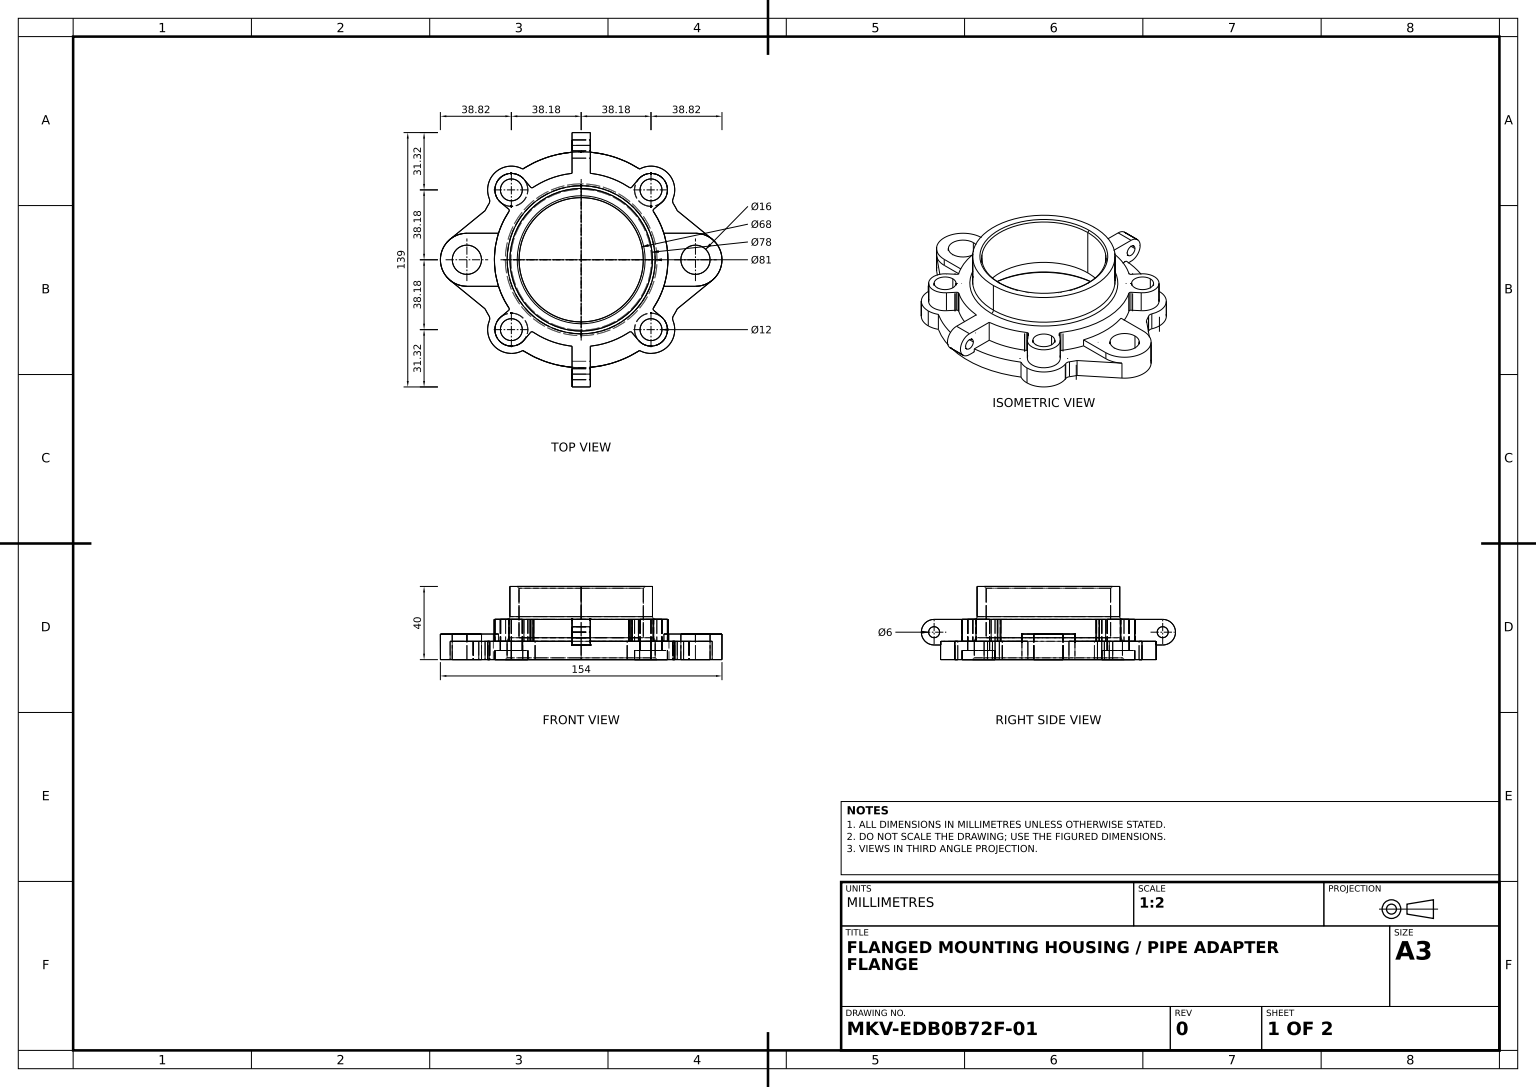
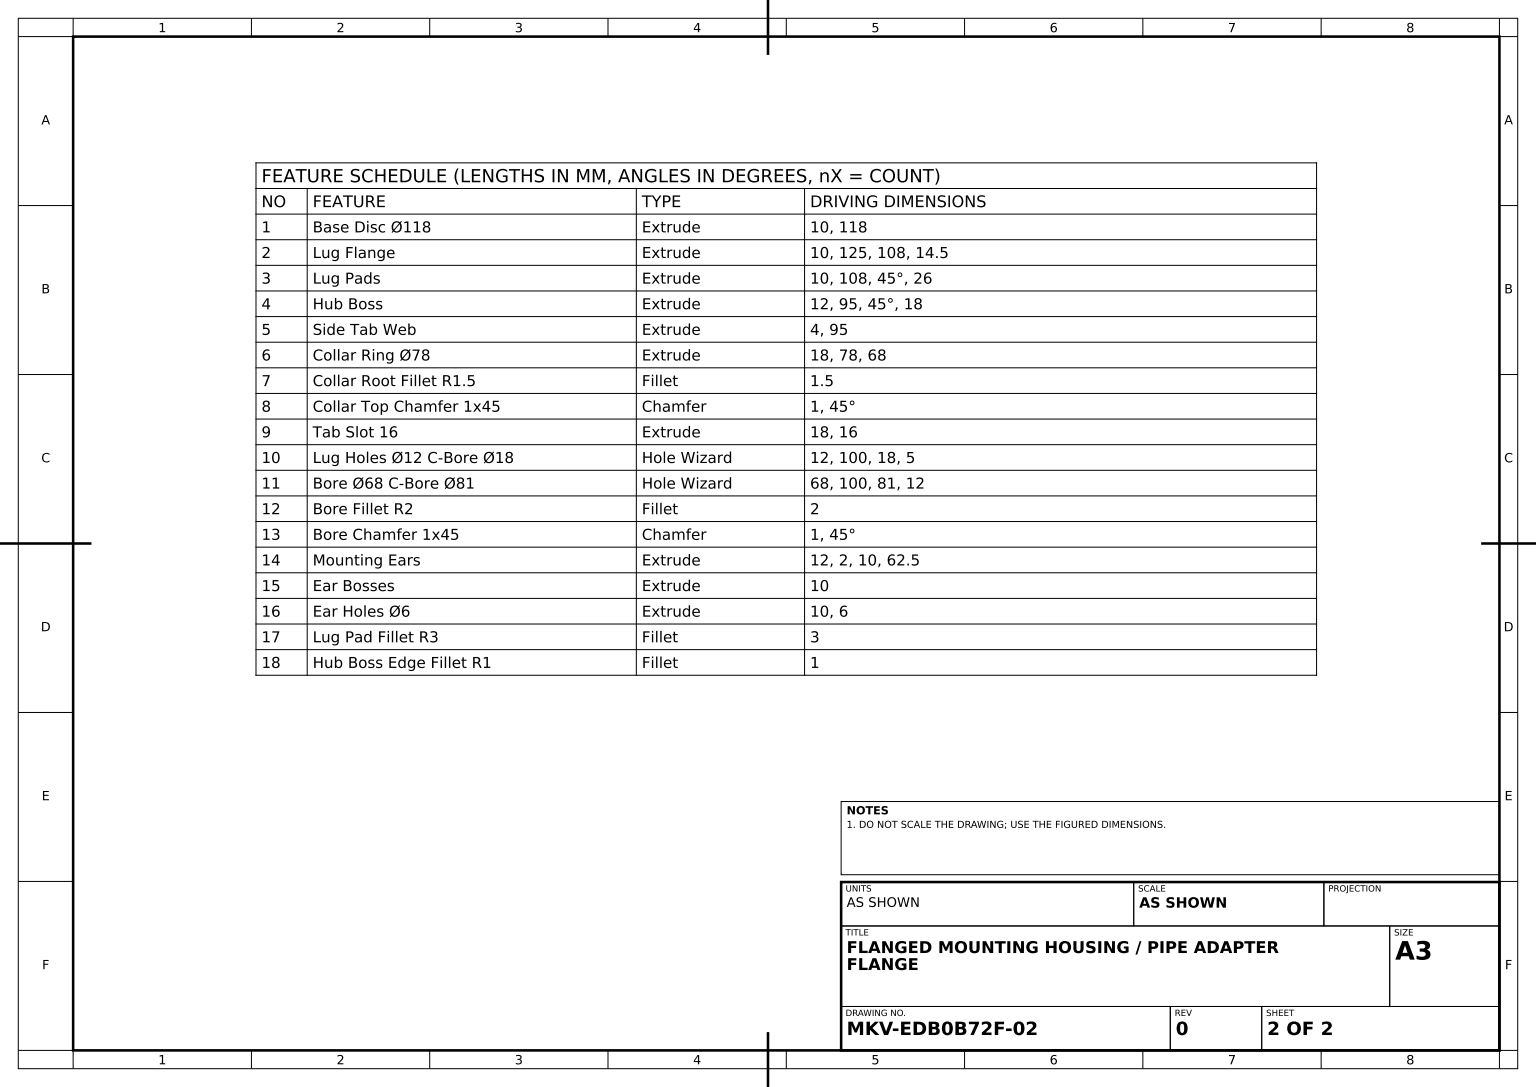
solid
v1 (-62.5,14,-14.5)
v2 (-62.5,10,-14.5)
e1 v1 v2 LINE
v3 (-45.232732,14,-14.5)
e2 v3 v1 LINE
v4 (-45.232732,10,-14.5)
e3 v3 v4 LINE
e4 v4 v2 LINE
face PLANE(AX(P(-62.5,14,-14.5),D(0,0,1),D(1,0,0))) rev [-e1 -e2 e3 e4]
v5 (5,8,-62.5)
v6 (5,15,-69.5)
e5 v5 v6 CIRCLE(AX(P(5,15,-62.5),D(1,0,0),D(0,0,-1)),7)
v7 (-5,8,-62.5)
e6 v5 v7 LINE
v8 (-5,15,-69.5)
e7 v7 v8 CIRCLE(AX(P(-5,15,-62.5),D(1,0,0),D(0,0,-1)),7)
e8 v8 v6 LINE
face CYL(AX(P(-5,15,-62.5),D(1,0,0),D(0,0,-1)),7) [-e5 e6 e7 e8]
v9 (71.664,10,-11.237042)
v10 (71.664,0,-11.237042)
e9 v9 v10 LINE
v11 (62.5,10,-14.5)
e10 v9 v11 CIRCLE(AX(P(62.5,10,0),D(0,1,0),D(0,0,-1)),14.5)
v12 (62.5,14,-14.5)
e11 v12 v11 LINE
v13 (62.5,14,14.5)
e12 v13 v12 CIRCLE(AX(P(62.5,14,0),D(0,1,0),D(0,0,-1)),14.5)
v14 (62.5,10,14.5)
e13 v13 v14 LINE
v15 (71.664,10,11.237042)
e14 v14 v15 CIRCLE(AX(P(62.5,10,0),D(0,1,0),D(0,0,-1)),14.5)
v16 (71.664,0,11.237042)
e15 v15 v16 LINE
e16 v10 v16 CIRCLE(AX(P(62.5,0,0),D(0,-1,0),D(0,0,-1)),14.5)
face CYL(AX(P(62.5,10,0),D(0,-1,0),D(0,0,-1)),14.5) [-e9 e10 -e11 -e12 e13 e14 e15 -e16]
v17 (45.232732,14,14.5)
e17 v17 v13 LINE
v18 (45.232732,10,14.5)
e18 v17 v18 LINE
e19 v18 v14 LINE
face PLANE(AX(P(62.5,14,14.5),D(0,0,-1),D(-1,0,0))) rev [-e13 -e17 e18 e19]
v19 (-38.183766,22,32.183766)
v20 (-38.183766,5,32.183766)
e20 v19 v20 LINE
v21 (-38.183766,5,44.183766)
e21 v20 v21 CIRCLE(AX(P(-38.183766,5,38.183766),D(0,-1,0),D(0,0,-1)),6)
v22 (-38.183766,22,44.183766)
e22 v22 v21 LINE
e23 v19 v22 CIRCLE(AX(P(-38.183766,22,38.183766),D(0,-1,0),D(0,0,-1)),6)
face CYL(AX(P(-38.183766,0,38.183766),D(0,-1,0),D(0,0,-1)),6) rev [e20 e21 -e22 -e23]
v23 (-5,8,58.787754)
v24 (-5,8,62.5)
e24 v23 v24 LINE
v25 (5,8,58.787754)
e25 v23 v25 CIRCLE(AX(P(0,8,0),D(0,1,0),D(0,0,1)),59)
v26 (5,8,62.5)
e26 v26 v25 LINE
e27 v24 v26 LINE
face PLANE(AX(P(0,8,0),D(0,1,0),D(0,0,1))) rev [-e24 e25 -e26 -e27]
v27 (-5,15,-59.5)
v28 (-5,15,-65.5)
e28 v27 v28 CIRCLE(AX(P(-5,15,-62.5),D(1,0,0),D(0,0,-1)),3)
v29 (5,15,-59.5)
e29 v27 v29 LINE
v30 (5,15,-65.5)
e30 v29 v30 CIRCLE(AX(P(5,15,-62.5),D(1,0,0),D(0,0,-1)),3)
e31 v28 v30 LINE
face CYL(AX(P(-5,15,-62.5),D(1,0,0),D(0,0,-1)),3) rev [-e28 e29 e30 -e31]
v31 (-50.441848,10,-30.604247)
v32 (-50.441848,0,-30.604247)
e32 v31 v32 LINE
v33 (-52.548788,0,-26.825824)
e33 v32 v33 CIRCLE(AX(P(0,0,0),D(0,1,0),D(0,0,1)),59)
v34 (-52.548788,10,-26.825824)
e34 v34 v33 LINE
e35 v31 v34 CIRCLE(AX(P(0,10,0),D(0,1,0),D(0,0,1)),59)
face CYL(AX(P(0,10,0),D(0,-1,0),D(0,0,-1)),59) [e32 e33 -e34 -e35]
v35 (-39.700135,10,27.679401)
v36 (-39.513984,10,26.360863)
e36 v35 v36 CIRCLE(AX(P(-40.345857,10,26.915829),D(0,1,0),D(0,0,1)),1)
v37 (-45.232732,10,14.5)
e37 v37 v36 CIRCLE(AX(P(0,10,0),D(0,1,0),D(0,0,1)),47.5)
v38 (-62.5,10,14.5)
e38 v38 v37 LINE
v39 (-71.664,10,11.237042)
e39 v39 v38 CIRCLE(AX(P(-62.5,10,0),D(0,1,0),D(0,0,1)),14.5)
v40 (-52.548788,10,26.825824)
e40 v40 v39 LINE
v41 (-50.441848,10,30.604247)
e41 v40 v41 CIRCLE(AX(P(0,10,0),D(0,1,0),D(0,0,1)),59)
v42 (-50.22739,10,33.289778)
e42 v41 v42 CIRCLE(AX(P(-53.006688,10,32.160396),D(0,-1,0),D(0,0,1)),3)
v43 (-38.183766,10,51.183766)
e43 v42 v43 CIRCLE(AX(P(-38.183766,10,38.183766),D(0,1,0),D(0,0,1)),13)
v44 (-31.95732,10,49.595662)
e44 v43 v44 CIRCLE(AX(P(-38.183766,10,38.183766),D(0,1,0),D(0,0,1)),13)
v45 (-5,10,58.787754)
e45 v44 v45 CIRCLE(AX(P(0,10,0),D(0,1,0),D(0,0,1)),59)
v46 (-5,10,47.236109)
e46 v46 v45 LINE
v47 (-26.360863,10,39.513984)
e47 v47 v46 CIRCLE(AX(P(0,10,0),D(0,1,0),D(0,0,1)),47.5)
v48 (-26.915829,10,39.345857)
e48 v47 v48 CIRCLE(AX(P(-26.915829,10,40.345857),D(0,1,0),D(0,0,1)),1)
v49 (-27.679401,10,39.700135)
e49 v48 v49 CIRCLE(AX(P(-26.915829,10,40.345857),D(0,1,0),D(0,0,1)),1)
v50 (-31.311611,10,43.995262)
e50 v50 v49 LINE
v51 (-43.995262,10,31.311611)
e51 v51 v50 CIRCLE(AX(P(-38.183766,10,38.183766),D(0,1,0),D(0,0,-1)),9)
e52 v35 v51 LINE
face PLANE(AX(P(0,10,0),D(0,1,0),D(0,0,1))) [e36 -e37 -e38 -e39 -e40 e41 e42 e43 e44 e45 -e46 -e47 e48 e49 -e50 -e51 -e52]
v52 (38.183766,5,-29.183766)
v53 (38.183766,5,-47.183766)
e53 v52 v53 CIRCLE(AX(P(38.183766,5,-38.183766),D(0,-1,0),D(0,0,-1)),9)
v54 (38.183766,0,-29.183766)
e54 v52 v54 LINE
v55 (38.183766,0,-47.183766)
e55 v54 v55 CIRCLE(AX(P(38.183766,0,-38.183766),D(0,-1,0),D(0,0,-1)),9)
e56 v53 v55 LINE
face CYL(AX(P(38.183766,0,-38.183766),D(0,-1,0),D(0,0,-1)),9) rev [-e53 e54 e55 -e56]
v56 (0,0,-59)
v57 (-31.95732,0,-49.595662)
e57 v56 v57 CIRCLE(AX(P(0,0,0),D(0,1,0),D(0,0,1)),59)
v58 (-31.95732,10,-49.595662)
e58 v57 v58 LINE
v59 (-5,10,-58.787754)
e59 v59 v58 CIRCLE(AX(P(0,10,0),D(0,1,0),D(0,0,1)),59)
v60 (-5,8,-58.787754)
e60 v59 v60 LINE
v61 (0,8,-59)
e61 v60 v61 CIRCLE(AX(P(0,8,0),D(0,-1,0),D(0,0,-1)),59)
e62 v61 v56 LINE
face CYL(AX(P(0,10,0),D(0,-1,0),D(0,0,-1)),59) [e57 e58 -e59 e60 e61 e62]
v62 (38.183766,22,-47.183766)
v63 (38.183766,10,-47.183766)
e63 v62 v63 LINE
v64 (43.995262,22,-31.311611)
e64 v64 v62 CIRCLE(AX(P(38.183766,22,-38.183766),D(0,1,0),D(0,0,-1)),9)
v65 (43.995262,10,-31.311611)
e65 v64 v65 LINE
e66 v65 v63 CIRCLE(AX(P(38.183766,10,-38.183766),D(0,1,0),D(0,0,-1)),9)
face CYL(AX(P(38.183766,22,-38.183766),D(0,-1,0),D(0,0,-1)),9) [-e63 -e64 e65 e66]
v66 (38.183766,5,29.183766)
v67 (38.183766,0,29.183766)
e67 v66 v67 LINE
v68 (38.183766,5,47.183766)
e68 v68 v66 CIRCLE(AX(P(38.183766,5,38.183766),D(0,-1,0),D(0,0,-1)),9)
v69 (38.183766,0,47.183766)
e69 v68 v69 LINE
e70 v69 v67 CIRCLE(AX(P(38.183766,0,38.183766),D(0,-1,0),D(0,0,-1)),9)
face CYL(AX(P(38.183766,0,38.183766),D(0,-1,0),D(0,0,-1)),9) rev [-e67 -e68 e69 e70]
v70 (-50.22739,0,33.289778)
e71 v42 v70 LINE
v71 (-50.441848,0,30.604247)
e72 v71 v41 LINE
e73 v70 v71 CIRCLE(AX(P(-53.006688,0,32.160396),D(0,1,0),D(0,0,1)),3)
face CYL(AX(P(-53.006688,0,32.160396),D(0,-1,0),D(0,0,-1)),3) rev [-e71 -e42 -e72 -e73]
v72 (-38.183766,22,-47.183766)
v73 (-38.183766,10,-47.183766)
e74 v72 v73 LINE
v74 (-31.311611,22,-43.995262)
e75 v74 v72 CIRCLE(AX(P(-38.183766,22,-38.183766),D(0,1,0),D(0,0,1)),9)
v75 (-31.311611,10,-43.995262)
e76 v74 v75 LINE
e77 v75 v73 CIRCLE(AX(P(-38.183766,10,-38.183766),D(0,1,0),D(0,0,1)),9)
face CYL(AX(P(-38.183766,22,-38.183766),D(0,-1,0),D(0,0,-1)),9) [-e74 -e75 e76 e77]
v76 (45.232732,10,-14.5)
v77 (39.513984,10,-26.360863)
e78 v76 v77 CIRCLE(AX(P(0,10,0),D(0,1,0),D(0,0,1)),47.5)
v78 (39.513984,22,-26.360863)
e79 v77 v78 LINE
v79 (39.513984,22,26.360863)
e80 v79 v78 CIRCLE(AX(P(0,22,0),D(0,1,0),D(0,0,1)),47.5)
v80 (39.513984,10,26.360863)
e81 v79 v80 LINE
e82 v80 v18 CIRCLE(AX(P(0,10,0),D(0,1,0),D(0,0,1)),47.5)
v81 (45.232732,14,-14.5)
e83 v81 v17 CIRCLE(AX(P(0,14,0),D(0,-1,0),D(0,0,-1)),47.5)
e84 v81 v76 LINE
face CYL(AX(P(0,22,0),D(0,-1,0),D(0,0,-1)),47.5) [e78 e79 -e80 e81 e82 -e18 -e83 e84]
v82 (0,40,39)
v83 (0,23.5,39)
e85 v82 v83 LINE
v84 (0,23.5,-39)
e86 v83 v84 CIRCLE(AX(P(0,23.5,0),D(0,1,0),D(0,0,-1)),39)
v85 (0,40,-39)
e87 v85 v84 LINE
e88 v82 v85 CIRCLE(AX(P(0,40,0),D(0,1,0),D(0,0,1)),39)
face CYL(AX(P(0,40,0),D(0,-1,0),D(0,0,-1)),39) [e85 e86 -e87 -e88]
v86 (-26.360863,22,39.513984)
e89 v86 v47 LINE
v87 (-26.915829,22,39.345857)
e90 v87 v86 CIRCLE(AX(P(-26.915829,22,40.345857),D(0,-1,0),D(0,0,-1)),1)
e91 v87 v48 LINE
face CYL(AX(P(-26.915829,22,40.345857),D(0,-1,0),D(0,0,-1)),1) rev [-e89 -e90 e91 -e48]
v88 (31.95732,0,-49.595662)
e92 v88 v56 CIRCLE(AX(P(0,0,0),D(0,1,0),D(0,0,1)),59)
v89 (5,8,-58.787754)
e93 v61 v89 CIRCLE(AX(P(0,8,0),D(0,-1,0),D(0,0,-1)),59)
v90 (5,10,-58.787754)
e94 v89 v90 LINE
v91 (31.95732,10,-49.595662)
e95 v91 v90 CIRCLE(AX(P(0,10,0),D(0,1,0),D(0,0,1)),59)
e96 v88 v91 LINE
face CYL(AX(P(0,10,0),D(0,-1,0),D(0,0,-1)),59) [e92 -e62 e93 e94 -e95 -e96]
e97 v7 v60 LINE
e98 v89 v5 LINE
face PLANE(AX(P(0,8,0),D(0,-1,0),D(0,0,-1))) [-e61 -e97 -e6 -e98 -e93]
v92 (-5,22,-62.5)
e99 v8 v92 CIRCLE(AX(P(-5,15,-62.5),D(1,0,0),D(0,0,-1)),7)
v93 (5,22,-62.5)
e100 v93 v92 LINE
e101 v6 v93 CIRCLE(AX(P(5,15,-62.5),D(1,0,0),D(0,0,-1)),7)
face CYL(AX(P(-5,15,-62.5),D(1,0,0),D(0,0,-1)),7) [e99 -e100 -e101 -e8]
v94 (0,22,40.5)
e102 v94 v83 CIRCLE(AX(P(0,23.5,40.5),D(1,0,0),D(0,0,-1)),1.5)
v95 (0,22,-40.5)
e103 v95 v94 CIRCLE(AX(P(0,22,0),D(0,-1,0),D(0,0,-1)),40.5)
e104 v95 v84 CIRCLE(AX(P(0,23.5,-40.5),D(-1,0,0),D(0,0,1)),1.5)
face TORUS(AX(P(0,23.5,0),D(0,-1,0),D(0,0,-1)),40.5,1.5) rev [-e86 -e102 -e103 e104]
v96 (52.548788,10,26.825824)
v97 (52.548788,0,26.825824)
e105 v96 v97 LINE
e106 v16 v97 LINE
e107 v15 v96 LINE
face PLANE(AX(P(71.664,10,11.237042),D(0.632,0,0.774968386),D(0.774968386,0,-0.632))) [e105 -e106 -e15 e107]
e108 v55 v54 CIRCLE(AX(P(38.183766,0,-38.183766),D(0,-1,0),D(0,0,-1)),9)
e109 v53 v52 CIRCLE(AX(P(38.183766,5,-38.183766),D(0,-1,0),D(0,0,-1)),9)
face CYL(AX(P(38.183766,0,-38.183766),D(0,-1,0),D(0,0,-1)),9) rev [e56 e108 -e54 -e109]
v98 (0,12,38.5)
v99 (0,12,-38.5)
e110 v98 v99 CIRCLE(AX(P(0,12,0),D(0,-1,0),D(0,0,1)),38.5)
e111 v99 v98 CIRCLE(AX(P(0,12,0),D(0,-1,0),D(0,0,1)),38.5)
v100 (0,12,-34)
v101 (0,12,34)
e112 v100 v101 CIRCLE(AX(P(0,12,0),D(0,-1,0),D(0,0,-1)),34)
e113 v101 v100 CIRCLE(AX(P(0,12,0),D(0,-1,0),D(0,0,-1)),34)
face PLANE(AX(P(34,12,0),D(0,1,0),D(0,0,1))) rev [e110 e111] [-e112 -e113]
v102 (-43.995262,22,-31.311611)
v103 (-39.700135,22,-27.679401)
e114 v102 v103 LINE
v104 (-43.995262,10,-31.311611)
e115 v102 v104 LINE
v105 (-39.700135,10,-27.679401)
e116 v104 v105 LINE
e117 v105 v103 LINE
face PLANE(AX(P(-43.995262,22,-31.311611),D(0.645721707,0,-0.763572837),D(-0.763572837,0,-0.645721707))) rev [-e114 e115 e116 e117]
v106 (-31.95732,0,49.595662)
e118 v106 v44 LINE
v107 (-38.183766,0,51.183766)
e119 v107 v43 LINE
e120 v107 v106 CIRCLE(AX(P(-38.183766,0,38.183766),D(0,1,0),D(0,0,1)),13)
face CYL(AX(P(-38.183766,0,38.183766),D(0,1,0),D(0,0,1)),13) [e118 -e44 -e119 e120]
v108 (50.441848,0,30.604247)
e121 v108 v97 CIRCLE(AX(P(0,0,0),D(0,1,0),D(0,0,1)),59)
v109 (50.441848,10,30.604247)
e122 v109 v96 CIRCLE(AX(P(0,10,0),D(0,1,0),D(0,0,1)),59)
e123 v109 v108 LINE
face CYL(AX(P(0,10,0),D(0,-1,0),D(0,0,-1)),59) [e121 -e105 -e122 e123]
v110 (52.548788,0,-26.825824)
e124 v110 v10 LINE
v111 (52.548788,10,-26.825824)
e125 v111 v110 LINE
e126 v111 v9 LINE
face PLANE(AX(P(71.664,10,-11.237042),D(0.632,0,-0.774968386),D(-0.774968386,0,-0.632))) [-e124 -e125 e126 e9]
v112 (-39.513984,10,-26.360863)
e127 v112 v4 CIRCLE(AX(P(0,10,0),D(0,1,0),D(0,0,1)),47.5)
e128 v112 v105 CIRCLE(AX(P(-40.345857,10,-26.915829),D(0,1,0),D(0,0,1)),1)
e129 v73 v104 CIRCLE(AX(P(-38.183766,10,-38.183766),D(0,1,0),D(0,0,1)),9)
v113 (-27.679401,10,-39.700135)
e130 v113 v75 LINE
v114 (-26.360863,10,-39.513984)
e131 v113 v114 CIRCLE(AX(P(-26.915829,10,-40.345857),D(0,1,0),D(0,0,1)),1)
v115 (-5,10,-47.236109)
e132 v115 v114 CIRCLE(AX(P(0,10,0),D(0,1,0),D(0,0,1)),47.5)
e133 v59 v115 LINE
v116 (-50.22739,10,-33.289778)
e134 v58 v116 CIRCLE(AX(P(-38.183766,10,-38.183766),D(0,1,0),D(0,0,-1)),13)
e135 v116 v31 CIRCLE(AX(P(-53.006688,10,-32.160396),D(0,-1,0),D(0,0,1)),3)
v117 (-71.664,10,-11.237042)
e136 v117 v34 LINE
e137 v2 v117 CIRCLE(AX(P(-62.5,10,0),D(0,1,0),D(0,0,1)),14.5)
face PLANE(AX(P(0,10,0),D(0,1,0),D(0,0,1))) [-e127 e128 -e116 -e129 -e77 -e130 e131 -e132 -e133 e59 e134 e135 e35 -e136 -e137 -e4]
v118 (-52.548788,0,26.825824)
e138 v40 v118 LINE
e139 v118 v71 CIRCLE(AX(P(0,0,0),D(0,1,0),D(0,0,1)),59)
face CYL(AX(P(0,10,0),D(0,-1,0),D(0,0,-1)),59) [-e41 e138 e139 e72]
v119 (0,10,-40.5)
e140 v119 v99 CIRCLE(AX(P(0,10,-38.5),D(1,0,0),D(0,0,-1)),2)
v120 (0,10,40.5)
e141 v120 v98 CIRCLE(AX(P(0,10,38.5),D(-1,0,0),D(0,0,1)),2)
e142 v119 v120 CIRCLE(AX(P(0,10,0),D(0,1,0),D(0,0,1)),40.5)
face TORUS(AX(P(0,10,0),D(0,1,0),D(0,0,1)),38.5,2) rev [e140 -e110 -e141 -e142]
v121 (-71.664,0,-11.237042)
e143 v117 v121 LINE
v122 (-71.664,0,11.237042)
e144 v122 v121 CIRCLE(AX(P(-62.5,0,0),D(0,-1,0),D(0,0,1)),14.5)
e145 v39 v122 LINE
v123 (-62.5,14,14.5)
e146 v123 v38 LINE
e147 v1 v123 CIRCLE(AX(P(-62.5,14,0),D(0,1,0),D(0,0,1)),14.5)
face CYL(AX(P(-62.5,10,0),D(0,-1,0),D(0,0,-1)),14.5) [e1 e137 e143 -e144 -e145 e39 -e146 -e147]
v124 (0,39,34)
v125 (0,40,35)
e148 v124 v125 LINE
v126 (0,40,-35)
e149 v126 v125 CIRCLE(AX(P(0,40,0),D(0,-1,0),D(0,0,1)),35)
v127 (0,39,-34)
e150 v127 v126 LINE
e151 v124 v127 CIRCLE(AX(P(0,39,0),D(0,1,0),D(0,0,1)),34)
face CONE(AX(P(0,39,0),D(0,1,0),D(0,0,1)),34,0.785398163) rev [e148 -e149 -e150 -e151]
v128 (50.22739,10,33.289778)
e152 v128 v109 CIRCLE(AX(P(53.006688,10,32.160396),D(0,-1,0),D(0,0,1)),3)
v129 (50.22739,0,33.289778)
e153 v129 v128 LINE
e154 v108 v129 CIRCLE(AX(P(53.006688,0,32.160396),D(0,1,0),D(0,0,1)),3)
face CYL(AX(P(53.006688,10,32.160396),D(0,-1,0),D(0,0,-1)),3) rev [-e123 -e152 -e153 -e154]
v130 (38.183766,22,-44.183766)
v131 (38.183766,22,-32.183766)
e155 v130 v131 CIRCLE(AX(P(38.183766,22,-38.183766),D(0,-1,0),D(0,0,-1)),6)
e156 v131 v130 CIRCLE(AX(P(38.183766,22,-38.183766),D(0,-1,0),D(0,0,-1)),6)
v132 (38.183766,22,44.183766)
v133 (38.183766,22,32.183766)
e157 v132 v133 CIRCLE(AX(P(38.183766,22,38.183766),D(0,-1,0),D(0,0,-1)),6)
e158 v133 v132 CIRCLE(AX(P(38.183766,22,38.183766),D(0,-1,0),D(0,0,-1)),6)
e159 v22 v19 CIRCLE(AX(P(-38.183766,22,38.183766),D(0,-1,0),D(0,0,-1)),6)
e160 v94 v95 CIRCLE(AX(P(0,22,0),D(0,-1,0),D(0,0,-1)),40.5)
v134 (-38.183766,22,-32.183766)
v135 (-38.183766,22,-44.183766)
e161 v134 v135 CIRCLE(AX(P(-38.183766,22,-38.183766),D(0,-1,0),D(0,0,-1)),6)
e162 v135 v134 CIRCLE(AX(P(-38.183766,22,-38.183766),D(0,-1,0),D(0,0,-1)),6)
v136 (-39.513984,22,-26.360863)
v137 (-39.513984,22,26.360863)
e163 v136 v137 CIRCLE(AX(P(0,22,0),D(0,1,0),D(0,0,1)),47.5)
v138 (-39.700135,22,27.679401)
e164 v137 v138 CIRCLE(AX(P(-40.345857,22,26.915829),D(0,-1,0),D(0,0,-1)),1)
v139 (-43.995262,22,31.311611)
e165 v138 v139 LINE
v140 (-31.311611,22,43.995262)
e166 v139 v140 CIRCLE(AX(P(-38.183766,22,38.183766),D(0,1,0),D(0,0,-1)),9)
v141 (-27.679401,22,39.700135)
e167 v140 v141 LINE
e168 v141 v87 CIRCLE(AX(P(-26.915829,22,40.345857),D(0,-1,0),D(0,0,-1)),1)
v142 (-5,22,47.236109)
e169 v86 v142 CIRCLE(AX(P(0,22,0),D(0,1,0),D(0,0,1)),47.5)
v143 (-5,22,62.5)
e170 v142 v143 LINE
v144 (5,22,62.5)
e171 v143 v144 LINE
v145 (5,22,47.236109)
e172 v144 v145 LINE
v146 (26.360863,22,39.513984)
e173 v145 v146 CIRCLE(AX(P(0,22,0),D(0,1,0),D(0,0,1)),47.5)
v147 (26.915829,22,39.345857)
e174 v146 v147 CIRCLE(AX(P(26.915829,22,40.345857),D(0,-1,0),D(0,0,-1)),1)
v148 (27.679401,22,39.700135)
e175 v147 v148 CIRCLE(AX(P(26.915829,22,40.345857),D(0,-1,0),D(0,0,-1)),1)
v149 (31.311611,22,43.995262)
e176 v148 v149 LINE
v150 (43.995262,22,31.311611)
e177 v149 v150 CIRCLE(AX(P(38.183766,22,38.183766),D(0,1,0),D(0,0,1)),9)
v151 (39.700135,22,27.679401)
e178 v150 v151 LINE
e179 v151 v79 CIRCLE(AX(P(40.345857,22,26.915829),D(0,-1,0),D(0,0,-1)),1)
v152 (39.700135,22,-27.679401)
e180 v78 v152 CIRCLE(AX(P(40.345857,22,-26.915829),D(0,-1,0),D(0,0,-1)),1)
e181 v152 v64 LINE
v153 (31.311611,22,-43.995262)
e182 v62 v153 CIRCLE(AX(P(38.183766,22,-38.183766),D(0,1,0),D(0,0,-1)),9)
v154 (27.679401,22,-39.700135)
e183 v153 v154 LINE
v155 (26.360863,22,-39.513984)
e184 v154 v155 CIRCLE(AX(P(26.915829,22,-40.345857),D(0,-1,0),D(0,0,-1)),1)
v156 (5,22,-47.236109)
e185 v155 v156 CIRCLE(AX(P(0,22,0),D(0,1,0),D(0,0,1)),47.5)
e186 v156 v93 LINE
v157 (-5,22,-47.236109)
e187 v92 v157 LINE
v158 (-26.360863,22,-39.513984)
e188 v157 v158 CIRCLE(AX(P(0,22,0),D(0,1,0),D(0,0,1)),47.5)
v159 (-27.679401,22,-39.700135)
e189 v158 v159 CIRCLE(AX(P(-26.915829,22,-40.345857),D(0,-1,0),D(0,0,-1)),1)
e190 v159 v74 LINE
e191 v72 v102 CIRCLE(AX(P(-38.183766,22,-38.183766),D(0,1,0),D(0,0,1)),9)
e192 v103 v136 CIRCLE(AX(P(-40.345857,22,-26.915829),D(0,-1,0),D(0,0,-1)),1)
face PLANE(AX(P(-38.183766,22,38.183766),D(0,-1,0),D(0,0,-1))) rev [e155 e156] [e157 e158] [e159 e23] [e160 e103] [e161 e162] [e163 e164 e165 e166 e167 e168 e90 e169 e170 e171 e172 e173 e174 e175 e176 e177 e178 e179 e80 e180 e181 e64 e182 e183 e184 e185 e186 e100 e187 e188 e189 e190 e75 e191 e114 e192]
e193 v36 v137 LINE
e194 v138 v35 LINE
face CYL(AX(P(-40.345857,22,26.915829),D(0,-1,0),D(0,0,-1)),1) rev [-e193 -e36 -e194 -e164]
v160 (38.183766,0,51.183766)
v161 (38.183766,10,51.183766)
e195 v160 v161 LINE
e196 v160 v129 CIRCLE(AX(P(38.183766,0,38.183766),D(0,1,0),D(0,0,-1)),13)
e197 v161 v128 CIRCLE(AX(P(38.183766,10,38.183766),D(0,1,0),D(0,0,-1)),13)
face CYL(AX(P(38.183766,0,38.183766),D(0,1,0),D(0,0,1)),13) [-e195 e196 e153 -e197]
v162 (-50.22739,0,-33.289778)
e198 v57 v162 CIRCLE(AX(P(-38.183766,0,-38.183766),D(0,1,0),D(0,0,-1)),13)
e199 v162 v116 LINE
face CYL(AX(P(-38.183766,0,-38.183766),D(0,1,0),D(0,0,1)),13) [-e58 e198 e199 -e134]
e200 v12 v81 LINE
e201 v11 v76 LINE
face PLANE(AX(P(62.5,14,-14.5),D(0,0,1),D(1,0,0))) rev [-e84 -e200 e11 e201]
v163 (-38.183766,5,29.183766)
v164 (-38.183766,0,29.183766)
e202 v163 v164 LINE
v165 (-38.183766,5,47.183766)
e203 v165 v163 CIRCLE(AX(P(-38.183766,5,38.183766),D(0,-1,0),D(0,0,-1)),9)
v166 (-38.183766,0,47.183766)
e204 v165 v166 LINE
e205 v166 v164 CIRCLE(AX(P(-38.183766,0,38.183766),D(0,-1,0),D(0,0,-1)),9)
face CYL(AX(P(-38.183766,0,38.183766),D(0,-1,0),D(0,0,-1)),9) rev [-e202 -e203 e204 e205]
v167 (26.360863,10,39.513984)
e206 v167 v146 LINE
v168 (26.915829,10,39.345857)
e207 v168 v167 CIRCLE(AX(P(26.915829,10,40.345857),D(0,1,0),D(0,0,1)),1)
e208 v147 v168 LINE
face CYL(AX(P(26.915829,22,40.345857),D(0,-1,0),D(0,0,-1)),1) rev [-e206 -e207 -e208 -e174]
e209 v143 v24 CIRCLE(AX(P(-5,15,62.5),D(1,0,0),D(0,0,-1)),7)
e210 v46 v142 LINE
e211 v23 v45 LINE
v169 (-5,15,59.5)
v170 (-5,15,65.5)
e212 v169 v170 CIRCLE(AX(P(-5,15,62.5),D(1,0,0),D(0,0,-1)),3)
e213 v170 v169 CIRCLE(AX(P(-5,15,62.5),D(1,0,0),D(0,0,-1)),3)
face PLANE(AX(P(-5,8,47.236109),D(-1,0,0),D(0,0,1))) [e24 -e209 -e170 -e210 e46 -e211] [e212 e213]
v171 (-45.232732,14,14.5)
e214 v171 v37 LINE
e215 v136 v112 LINE
e216 v171 v3 CIRCLE(AX(P(0,14,0),D(0,-1,0),D(0,0,-1)),47.5)
face CYL(AX(P(0,22,0),D(0,-1,0),D(0,0,-1)),47.5) [e214 e37 e193 -e163 e215 e127 -e3 -e216]
v172 (39.700135,10,-27.679401)
e217 v172 v65 LINE
e218 v152 v172 LINE
face PLANE(AX(P(43.995262,22,-31.311611),D(-0.645721707,0,-0.763572837),D(-0.763572837,0,0.645721707))) rev [e217 -e65 -e181 e218]
v173 (50.441848,0,-30.604247)
v174 (50.441848,10,-30.604247)
e219 v173 v174 LINE
v175 (50.22739,0,-33.289778)
e220 v175 v173 CIRCLE(AX(P(53.006688,0,-32.160396),D(0,1,0),D(0,0,1)),3)
v176 (50.22739,10,-33.289778)
e221 v176 v175 LINE
e222 v174 v176 CIRCLE(AX(P(53.006688,10,-32.160396),D(0,-1,0),D(0,0,1)),3)
face CYL(AX(P(53.006688,0,-32.160396),D(0,-1,0),D(0,0,-1)),3) rev [-e219 -e220 -e221 -e222]
v177 (-38.183766,0,-29.183766)
v178 (-38.183766,0,-47.183766)
e223 v177 v178 CIRCLE(AX(P(-38.183766,0,-38.183766),D(0,-1,0),D(0,0,-1)),9)
v179 (-38.183766,5,-47.183766)
e224 v179 v178 LINE
v180 (-38.183766,5,-29.183766)
e225 v180 v179 CIRCLE(AX(P(-38.183766,5,-38.183766),D(0,-1,0),D(0,0,-1)),9)
e226 v180 v177 LINE
face CYL(AX(P(-38.183766,0,-38.183766),D(0,-1,0),D(0,0,-1)),9) rev [e223 -e224 -e225 e226]
e227 v172 v77 CIRCLE(AX(P(40.345857,10,-26.915829),D(0,1,0),D(0,0,1)),1)
face CYL(AX(P(40.345857,22,-26.915829),D(0,-1,0),D(0,0,-1)),1) rev [-e79 -e227 -e218 -e180]
v181 (0,1,40.5)
v182 (0,0,41.5)
e228 v181 v182 LINE
v183 (0,0,-41.5)
e229 v183 v182 CIRCLE(AX(P(0,0,0),D(0,1,0),D(0,0,1)),41.5)
v184 (0,1,-40.5)
e230 v184 v183 LINE
e231 v181 v184 CIRCLE(AX(P(0,1,0),D(0,-1,0),D(0,0,1)),40.5)
face CONE(AX(P(0,1,0),D(0,-1,0),D(0,0,-1)),40.5,0.785398163) rev [e228 -e229 -e230 -e231]
e232 v139 v51 LINE
face PLANE(AX(P(-43.995262,22,31.311611),D(0.645721707,0,0.763572837),D(0.763572837,0,-0.645721707))) rev [e52 -e232 -e165 e194]
v185 (-62.5,14,8)
v186 (-62.5,14,-8)
e233 v185 v186 CIRCLE(AX(P(-62.5,14,0),D(0,1,0),D(0,0,1)),8)
v187 (-62.5,0,-8)
e234 v187 v186 LINE
v188 (-62.5,0,8)
e235 v188 v187 CIRCLE(AX(P(-62.5,0,0),D(0,1,0),D(0,0,1)),8)
e236 v188 v185 LINE
face CYL(AX(P(-62.5,-4,0),D(0,1,0),D(0,0,1)),8) rev [e233 -e234 -e235 e236]
e237 v175 v88 CIRCLE(AX(P(38.183766,0,-38.183766),D(0,1,0),D(0,0,1)),13)
e238 v176 v91 CIRCLE(AX(P(38.183766,10,-38.183766),D(0,1,0),D(0,0,1)),13)
face CYL(AX(P(38.183766,0,-38.183766),D(0,1,0),D(0,0,1)),13) [e237 e96 -e238 e221]
v189 (38.183766,5,32.183766)
e239 v133 v189 LINE
v190 (38.183766,5,44.183766)
e240 v189 v190 CIRCLE(AX(P(38.183766,5,38.183766),D(0,-1,0),D(0,0,-1)),6)
e241 v132 v190 LINE
face CYL(AX(P(38.183766,0,38.183766),D(0,-1,0),D(0,0,-1)),6) rev [e239 e240 -e241 -e158]
e242 v178 v177 CIRCLE(AX(P(-38.183766,0,-38.183766),D(0,-1,0),D(0,0,-1)),9)
e243 v179 v180 CIRCLE(AX(P(-38.183766,5,-38.183766),D(0,-1,0),D(0,0,-1)),9)
face CYL(AX(P(-38.183766,0,-38.183766),D(0,-1,0),D(0,0,-1)),9) rev [e242 -e226 -e243 e224]
e244 v85 v82 CIRCLE(AX(P(0,40,0),D(0,1,0),D(0,0,1)),39)
e245 v84 v83 CIRCLE(AX(P(0,23.5,0),D(0,1,0),D(0,0,-1)),39)
face CYL(AX(P(0,40,0),D(0,-1,0),D(0,0,-1)),39) [-e85 -e244 e87 e245]
v191 (5,15,59.5)
e246 v169 v191 LINE
v192 (5,15,65.5)
e247 v170 v192 LINE
e248 v192 v191 CIRCLE(AX(P(5,15,62.5),D(1,0,0),D(0,0,-1)),3)
face CYL(AX(P(-5,15,62.5),D(1,0,0),D(0,0,-1)),3) rev [-e246 -e213 e247 e248]
e249 v28 v27 CIRCLE(AX(P(-5,15,-62.5),D(1,0,0),D(0,0,-1)),3)
e250 v115 v157 LINE
face PLANE(AX(P(-5,8,-47.236109),D(-1,0,0),D(0,0,1))) [e28 e249] [e97 -e60 e133 e250 -e187 -e99 -e7]
e251 v111 v174 CIRCLE(AX(P(0,10,0),D(0,1,0),D(0,0,1)),59)
e252 v110 v173 CIRCLE(AX(P(0,0,0),D(0,1,0),D(0,0,1)),59)
face CYL(AX(P(0,10,0),D(0,-1,0),D(0,0,-1)),59) [-e251 e125 e252 e219]
v193 (27.679401,10,39.700135)
e253 v193 v168 CIRCLE(AX(P(26.915829,10,40.345857),D(0,1,0),D(0,0,1)),1)
e254 v148 v193 LINE
face CYL(AX(P(26.915829,22,40.345857),D(0,-1,0),D(0,0,-1)),1) rev [-e175 e208 -e253 -e254]
v194 (43.995262,10,31.311611)
e255 v150 v194 LINE
v195 (31.311611,10,43.995262)
e256 v149 v195 LINE
e257 v195 v194 CIRCLE(AX(P(38.183766,10,38.183766),D(0,1,0),D(0,0,1)),9)
face CYL(AX(P(38.183766,22,38.183766),D(0,-1,0),D(0,0,-1)),9) [-e255 -e177 e256 e257]
e258 v120 v119 CIRCLE(AX(P(0,10,0),D(0,1,0),D(0,0,1)),40.5)
face TORUS(AX(P(0,10,0),D(0,1,0),D(0,0,1)),38.5,2) rev [-e140 -e258 e141 -e111]
e259 v125 v126 CIRCLE(AX(P(0,40,0),D(0,-1,0),D(0,0,1)),35)
face PLANE(AX(P(0,40,0),D(0,1,0),D(0,0,1))) [e88 e244] [e259 e149]
v196 (-38.183766,5,-32.183766)
v197 (-38.183766,5,-44.183766)
e260 v196 v197 CIRCLE(AX(P(-38.183766,5,-38.183766),D(0,-1,0),D(0,0,-1)),6)
e261 v197 v196 CIRCLE(AX(P(-38.183766,5,-38.183766),D(0,-1,0),D(0,0,-1)),6)
face PLANE(AX(P(-32.183766,5,-38.183766),D(0,1,0),D(0,0,1))) rev [-e260 -e261] [e225 e243]
e262 v127 v124 CIRCLE(AX(P(0,39,0),D(0,1,0),D(0,0,1)),34)
face CONE(AX(P(0,39,0),D(0,1,0),D(0,0,1)),34,0.785398163) rev [-e148 -e262 e150 -e259]
v198 (31.311611,10,-43.995262)
v199 (27.679401,10,-39.700135)
e263 v198 v199 LINE
e264 v199 v154 LINE
e265 v153 v198 LINE
face PLANE(AX(P(31.311611,22,-43.995262),D(0.763572837,0,0.645721707),D(0.645721707,0,-0.763572837))) rev [e263 e264 -e183 e265]
e266 v124 v101 LINE
e267 v127 v100 LINE
face CYL(AX(P(0,40,0),D(0,-1,0),D(0,0,-1)),34) rev [e112 -e266 e151 e267]
e268 v144 v26 CIRCLE(AX(P(5,15,62.5),D(1,0,0),D(0,0,-1)),7)
face CYL(AX(P(-5,15,62.5),D(1,0,0),D(0,0,-1)),7) [e27 -e268 -e171 e209]
e269 v135 v197 LINE
e270 v134 v196 LINE
face CYL(AX(P(-38.183766,0,-38.183766),D(0,-1,0),D(0,0,-1)),6) rev [-e162 e269 e261 -e270]
e271 v63 v198 CIRCLE(AX(P(38.183766,10,-38.183766),D(0,1,0),D(0,0,-1)),9)
face CYL(AX(P(38.183766,22,-38.183766),D(0,-1,0),D(0,0,-1)),9) [e63 e271 -e265 -e182]
e272 v49 v141 LINE
face CYL(AX(P(-26.915829,22,40.345857),D(0,-1,0),D(0,0,-1)),1) rev [-e272 -e49 -e91 -e168]
e273 v164 v166 CIRCLE(AX(P(-38.183766,0,38.183766),D(0,-1,0),D(0,0,-1)),9)
v200 (62.5,0,8)
v201 (62.5,0,-8)
e274 v200 v201 CIRCLE(AX(P(62.5,0,0),D(0,1,0),D(0,0,1)),8)
e275 v201 v200 CIRCLE(AX(P(62.5,0,0),D(0,1,0),D(0,0,1)),8)
e276 v182 v183 CIRCLE(AX(P(0,0,0),D(0,1,0),D(0,0,1)),41.5)
e277 v67 v69 CIRCLE(AX(P(38.183766,0,38.183766),D(0,-1,0),D(0,0,-1)),9)
v202 (31.95732,0,49.595662)
e278 v202 v160 CIRCLE(AX(P(38.183766,0,38.183766),D(0,1,0),D(0,0,-1)),13)
e279 v106 v202 CIRCLE(AX(P(0,0,0),D(0,1,0),D(0,0,1)),59)
e280 v70 v107 CIRCLE(AX(P(-38.183766,0,38.183766),D(0,1,0),D(0,0,1)),13)
e281 v118 v122 LINE
e282 v121 v33 LINE
e283 v32 v162 CIRCLE(AX(P(-53.006688,0,-32.160396),D(0,1,0),D(0,0,1)),3)
e284 v187 v188 CIRCLE(AX(P(-62.5,0,0),D(0,1,0),D(0,0,1)),8)
face PLANE(AX(P(0,0,0),D(0,1,0),D(0,0,1))) rev [-e205 -e273] [-e242 -e223] [e274 e275] [e229 e276] [-e70 -e277] [-e121 e154 -e196 -e278 -e279 -e120 -e280 e73 -e139 e281 e144 e282 -e33 e283 -e198 -e57 -e92 -e237 e220 -e252 e124 e16 e106] [e235 e284] [-e108 -e55]
e285 v120 v181 LINE
e286 v119 v184 LINE
face CYL(AX(P(0,0,0),D(0,-1,0),D(0,0,-1)),40.5) rev [e142 e285 e231 -e286]
face CYL(AX(P(-38.183766,0,-38.183766),D(0,-1,0),D(0,0,-1)),6) rev [-e269 -e161 e270 e260]
e287 v123 v171 LINE
e288 v186 v185 CIRCLE(AX(P(-62.5,14,0),D(0,1,0),D(0,0,1)),8)
face PLANE(AX(P(62.5,14,0),D(0,-1,0),D(0,0,-1))) rev [e287 e216 e2 e147] [-e288 -e233]
face CYL(AX(P(-62.5,-4,0),D(0,1,0),D(0,0,1)),8) rev [e288 -e236 -e284 e234]
e289 v30 v29 CIRCLE(AX(P(5,15,-62.5),D(1,0,0),D(0,0,-1)),3)
face CYL(AX(P(-5,15,-62.5),D(1,0,0),D(0,0,-1)),3) rev [-e249 e31 e289 -e29]
e290 v190 v189 CIRCLE(AX(P(38.183766,5,38.183766),D(0,-1,0),D(0,0,-1)),6)
e291 v66 v68 CIRCLE(AX(P(38.183766,5,38.183766),D(0,-1,0),D(0,0,-1)),9)
face PLANE(AX(P(44.183766,5,38.183766),D(0,1,0),D(0,0,1))) rev [-e240 -e290] [e291 e68]
e292 v21 v20 CIRCLE(AX(P(-38.183766,5,38.183766),D(0,-1,0),D(0,0,-1)),6)
e293 v163 v165 CIRCLE(AX(P(-38.183766,5,38.183766),D(0,-1,0),D(0,0,-1)),9)
face PLANE(AX(P(-32.183766,5,38.183766),D(0,1,0),D(0,0,1))) rev [-e292 -e21] [e293 e203]
face CYL(AX(P(0,40,0),D(0,-1,0),D(0,0,-1)),34) rev [-e267 e262 e266 e113]
e294 v184 v181 CIRCLE(AX(P(0,1,0),D(0,-1,0),D(0,0,1)),40.5)
face CYL(AX(P(0,0,0),D(0,-1,0),D(0,0,-1)),40.5) rev [e294 -e285 e258 e286]
e295 v191 v192 CIRCLE(AX(P(5,15,62.5),D(1,0,0),D(0,0,-1)),3)
face CYL(AX(P(-5,15,62.5),D(1,0,0),D(0,0,-1)),3) rev [e295 -e247 -e212 e246]
face CYL(AX(P(-38.183766,0,38.183766),D(0,1,0),D(0,0,1)),13) [e71 e280 e119 -e43]
face PLANE(AX(P(-71.664,10,-11.237042),D(-0.632,0,-0.774968386),D(-0.774968386,0,0.632))) [-e282 -e143 e136 e34]
v203 (31.95732,10,49.595662)
e296 v202 v203 LINE
v204 (5,10,58.787754)
e297 v204 v203 CIRCLE(AX(P(0,10,0),D(0,1,0),D(0,0,1)),59)
e298 v204 v25 LINE
face CYL(AX(P(0,10,0),D(0,-1,0),D(0,0,-1)),59) [e279 e296 -e297 e298 -e25 e211 -e45 -e118]
face CYL(AX(P(-38.183766,22,-38.183766),D(0,-1,0),D(0,0,-1)),9) [-e191 e74 e129 -e115]
e299 v114 v158 LINE
face CYL(AX(P(0,22,0),D(0,-1,0),D(0,0,-1)),47.5) [-e188 -e250 e132 e299]
face CYL(AX(P(38.183766,0,38.183766),D(0,-1,0),D(0,0,-1)),6) rev [e290 -e239 -e157 e241]
v205 (62.5,14,-8)
v206 (62.5,14,8)
e300 v205 v206 CIRCLE(AX(P(62.5,14,0),D(0,1,0),D(0,0,1)),8)
e301 v206 v205 CIRCLE(AX(P(62.5,14,0),D(0,1,0),D(0,0,1)),8)
face PLANE(AX(P(62.5,14,0),D(0,-1,0),D(0,0,-1))) rev [-e300 -e301] [e83 e17 e12 e200]
face PLANE(AX(P(-62.5,14,14.5),D(0,0,-1),D(-1,0,0))) rev [e146 e38 -e214 -e287]
v207 (5,10,47.236109)
e302 v207 v167 CIRCLE(AX(P(0,10,0),D(0,1,0),D(0,0,1)),47.5)
e303 v204 v207 LINE
e304 v203 v161 CIRCLE(AX(P(38.183766,10,38.183766),D(0,1,0),D(0,0,-1)),13)
v208 (39.700135,10,27.679401)
e305 v80 v208 CIRCLE(AX(P(40.345857,10,26.915829),D(0,1,0),D(0,0,1)),1)
e306 v194 v208 LINE
e307 v193 v195 LINE
face PLANE(AX(P(0,10,0),D(0,1,0),D(0,0,1))) [e253 e207 -e302 -e303 e297 e304 e197 e152 e122 -e107 -e14 -e19 -e82 e305 -e306 -e257 -e307]
e308 v207 v145 LINE
face PLANE(AX(P(5,8,47.236109),D(1,0,0),D(0,0,-1))) [-e248 -e295] [e303 e308 -e172 e268 e26 -e298]
e309 v159 v113 LINE
face CYL(AX(P(-26.915829,22,-40.345857),D(0,-1,0),D(0,0,-1)),1) rev [-e131 -e309 -e189 -e299]
face CONE(AX(P(0,1,0),D(0,-1,0),D(0,0,-1)),40.5,0.785398163) rev [-e276 -e228 -e294 e230]
face PLANE(AX(P(31.311611,22,43.995262),D(0.763572837,0,-0.645721707),D(-0.645721707,0,-0.763572837))) rev [e254 e307 -e256 -e176]
v209 (26.360863,10,-39.513984)
v210 (5,10,-47.236109)
e310 v209 v210 CIRCLE(AX(P(0,10,0),D(0,1,0),D(0,0,1)),47.5)
e311 v209 v199 CIRCLE(AX(P(26.915829,10,-40.345857),D(0,1,0),D(0,0,1)),1)
e312 v210 v90 LINE
face PLANE(AX(P(0,10,0),D(0,1,0),D(0,0,1))) [-e310 e311 -e263 -e271 -e66 -e217 e227 -e78 -e201 -e10 -e126 e251 e222 e238 e95 -e312]
face CYL(AX(P(38.183766,0,38.183766),D(0,1,0),D(0,0,1)),13) [-e304 -e296 e278 e195]
v211 (38.183766,5,-44.183766)
v212 (38.183766,5,-32.183766)
e313 v211 v212 CIRCLE(AX(P(38.183766,5,-38.183766),D(0,-1,0),D(0,0,-1)),6)
e314 v212 v211 CIRCLE(AX(P(38.183766,5,-38.183766),D(0,-1,0),D(0,0,-1)),6)
face PLANE(AX(P(44.183766,5,-38.183766),D(0,1,0),D(0,0,1))) rev [-e313 -e314] [e109 e53]
face CYL(AX(P(-38.183766,0,38.183766),D(0,-1,0),D(0,0,-1)),9) rev [-e204 -e293 e202 e273]
e315 v140 v50 LINE
face PLANE(AX(P(-31.311611,22,43.995262),D(-0.763572837,0,-0.645721707),D(-0.645721707,0,0.763572837))) rev [e315 e50 e272 -e167]
e316 v200 v206 LINE
e317 v201 v205 LINE
face CYL(AX(P(62.5,-4,0),D(0,1,0),D(0,0,1)),8) rev [e316 e301 -e317 -e274]
face CYL(AX(P(-38.183766,0,38.183766),D(0,-1,0),D(0,0,-1)),6) rev [-e159 e22 e292 -e20]
face CYL(AX(P(38.183766,0,38.183766),D(0,-1,0),D(0,0,-1)),9) rev [e67 e277 -e69 -e291]
e318 v155 v209 LINE
face CYL(AX(P(26.915829,22,-40.345857),D(0,-1,0),D(0,0,-1)),1) rev [-e318 -e184 -e264 -e311]
face CYL(AX(P(0,22,0),D(0,-1,0),D(0,0,-1)),47.5) [-e173 -e308 e302 e206]
face PLANE(AX(P(-71.664,10,11.237042),D(-0.632,0,0.774968386),D(0.774968386,0,0.632))) [-e281 -e138 e40 e145]
e319 v210 v156 LINE
face PLANE(AX(P(5,8,-47.236109),D(1,0,0),D(0,0,-1))) [-e186 -e319 e312 -e94 e98 e5 e101] [-e289 -e30]
face CYL(AX(P(-38.183766,22,38.183766),D(0,-1,0),D(0,0,-1)),9) [e232 e51 -e315 -e166]
face CYL(AX(P(0,22,0),D(0,-1,0),D(0,0,-1)),47.5) [e47 e210 -e169 e89]
face CYL(AX(P(-40.345857,22,-26.915829),D(0,-1,0),D(0,0,-1)),1) rev [-e215 -e192 -e117 -e128]
e320 v130 v211 LINE
e321 v131 v212 LINE
face CYL(AX(P(38.183766,0,-38.183766),D(0,-1,0),D(0,0,-1)),6) rev [-e155 e320 e313 -e321]
face PLANE(AX(P(-31.311611,22,-43.995262),D(-0.763572837,0,0.645721707),D(0.645721707,0,0.763572837))) rev [-e76 -e190 e309 e130]
face CYL(AX(P(38.183766,0,-38.183766),D(0,-1,0),D(0,0,-1)),6) rev [e314 -e320 -e156 e321]
e322 v208 v151 LINE
face PLANE(AX(P(43.995262,22,31.311611),D(-0.645721707,0,0.763572837),D(0.763572837,0,0.645721707))) rev [e255 e306 e322 -e178]
face CYL(AX(P(0,22,0),D(0,-1,0),D(0,0,-1)),47.5) [-e185 e318 e310 e319]
face TORUS(AX(P(0,23.5,0),D(0,-1,0),D(0,0,-1)),40.5,1.5) rev [-e160 e102 -e245 -e104]
face CYL(AX(P(-53.006688,10,-32.160396),D(0,-1,0),D(0,0,-1)),3) rev [-e199 -e283 -e32 -e135]
face CYL(AX(P(62.5,-4,0),D(0,1,0),D(0,0,1)),8) rev [-e275 e317 e300 -e316]
face CYL(AX(P(40.345857,22,26.915829),D(0,-1,0),D(0,0,-1)),1) rev [-e305 -e81 -e179 -e322]
